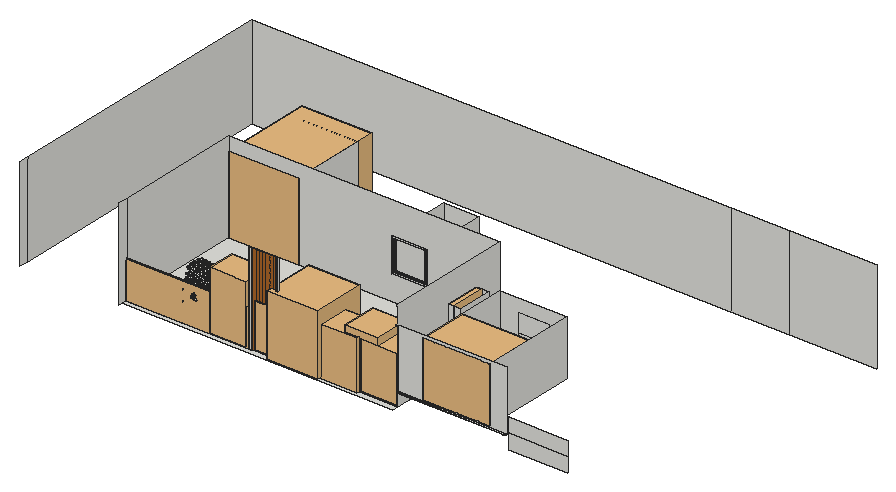
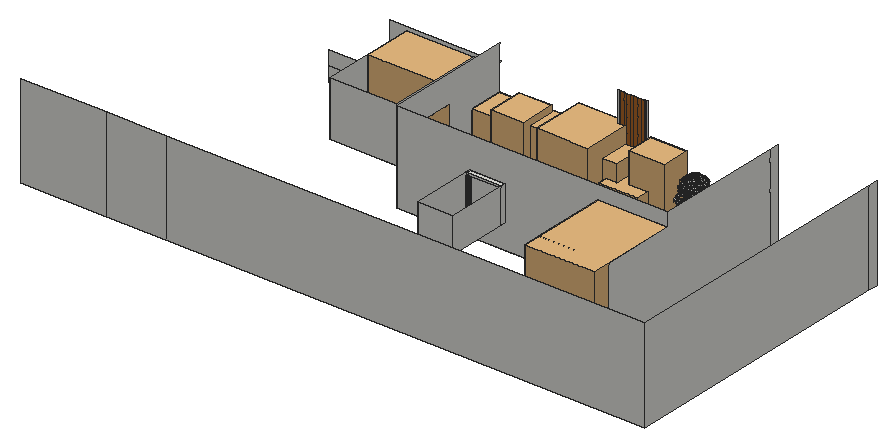
# SketchUp Ruby script. Lengths in inches.
U = 1.inch
M = Sketchup.active_model
def pt(a) = Geom::Point3d.new(a.map { |v| v * U })
def face(e, loops, mat)
  f = e.add_face(loops[0].map { |a| pt(a) })
  loops[1..].each { |l| e.add_face(l.map { |a| pt(a) }).erase! }
  f.material = f.back_material = mat if mat
  f
end
# faces: each face lists its corners as indices into pts; further lists are holes
def faces(e, pts, list, mat = nil) = list.each { |f| face(e, (f[0].is_a?(Array) ? f : [f]).map { |l| l.map { |i| pts[i] } }, mat) }
# xy, xz, yz: faces in a plane at the given z, y or x. An outline is a flat list of corners, or four numbers for a rectangle; further outlines are holes
def ring(l) = l.size == 4 ? [[l[0], l[1]], [l[2], l[1]], [l[2], l[3]], [l[0], l[3]]] : l.each_slice(2).to_a
def flat(e, list, mat, &to3) = list.each { |f| face(e, (f[0].is_a?(Array) ? f : [f]).map { |l| ring(l).map { |u, v| to3.(u, v) } }, mat) }
def xy(e, z, list, mat = nil) = flat(e, list, mat) { |x, y| [x, y, z] }
def xz(e, y, list, mat = nil) = flat(e, list, mat) { |x, z| [x, y, z] }
def yz(e, x, list, mat = nil) = flat(e, list, mat) { |y, z| [x, y, z] }
def lines(e, pts, list) = list.each { |a, b| e.add_line(pt(pts[a]), pt(pts[b])) }
# prism: a flat outline (further loops are holes) pulled along v
def prism(e, loops, v, mat = nil)
  f = face(e, loops, mat); d = Geom::Vector3d.new(v.map { |x| x * U })
  f.pushpull(f.normal.samedirection?(d) ? d.length : -d.length)
end
def box(e, o, s, mat = nil) = prism(e, [[o, [o[0] + s[0], o[1], o[2]], [o[0] + s[0], o[1] + s[1], o[2]], [o[0], o[1] + s[1], o[2]]]], [0, 0, s[2]], mat)
def at(x, y, z, deg = 0) = Geom::Transformation.translation(pt([x, y, z])) * Geom::Transformation.rotation(ORIGIN, Z_AXIS, deg.degrees)
def axes(o, x, y, z) = Geom::Transformation.new([*x, 0, *y, 0, *z, 0, *pt(o).to_a, 1])
def part(name) = M.definitions.add(name)
# library, detail: a bought-in or finely detailed component or shape, given as its bounding box
def library(name, o, s) = part(name).tap { |d| box(d.entities, o, s) }
def detail(e, o, s) = box(e.add_group.entities, o, s)
def put(e, d, t, mat = nil) = e.add_instance(d, t).tap { |i| i.material = mat if mat }
def group(e, t, mat = nil) = e.add_group.tap { |g| g.transformation = t; g.material = mat if mat }.entities
root = M.entities
M.materials.add("[Wood Bamboo]").color = [173, 103, 41]
c1 = library("Glass Railings(black Handrails)",[-57.04,-132.55,0],[169.29,2.52,28.17])
c2 = library("Hanging Plant\#2",[-3.24,-1.74,-0.87],[34.15,22.4,50.98])
c3 = library("Yukka Plant GHD",[0,0,0],[46.13,35.26,75.51])
c4 = library("Philodendron Plant GHD",[-18.43,-10.97,-1.09],[51.75,39.48,62.43])
c5 = library("Plant Banana",[3.49,5.74,0],[38.27,39.55,56.51])
c6 = library("Potted indoor plant",[-35.72,-28.42,0],[66.31,67.39,78.4375])
c7 = part("leaflet")
p = [[2.87,10.24,0.32],[0.33,13.79,0],[-2.24,10.39,0.32],[-2.2,6.92,0.33],[0.45,0.11,0.33],[2.91,6.86,0.33]]
faces(c7.entities,p,[[0,1,2],[0,2,3,4,5]])
c8 = part("leaf group")
put(c8.entities,c7,axes([4.25,4.04,0.04],[0.8,0,0],[0,0.8,0],[0,0,0.8]))
put(c8.entities,c7,axes([4.5,3.78,0.04],[0.4,0.69282,-0.00011],[-0.69282,0.4,-0.00008],[-0.00001,0.00014,0.8]))
put(c8.entities,c7,axes([4.92,3.9375,0.04],[-0.56569,0.56569,-0.00025],[-0.56569,-0.56569,0.00001],[-0.00017,0.00019,0.8]))
put(c8.entities,c7,axes([4.87,4.38,0.04],[-0.69282,-0.4,-0.0002],[0.4,-0.69282,0.00017],[-0.00026,0.00005,0.8]))
put(c8.entities,c7,axes([4.42,4.45,0.04],[0.20706,-0.77274,-0.00003],[0.77274,0.20706,0.00016],[-0.00015,-0.00007,0.8]))
c9 = part("branch with leaves\#1")
put(c9.entities,c8,axes([2.86,31.23,35.15],[-0.02765,-0.79009,-0.61237],[0.48114,-0.54749,0.68465],[-0.8762,-0.27571,0.39528]))
put(c9.entities,c8,axes([12.72,29.5,24.05],[-0.41566,0.90952,0],[-0.44736,-0.20444,-0.87067],[-0.7919,-0.3619,0.49186]))
put(c9.entities,c8,axes([15.91,15.09,15.29],[-0.51919,0.82474,-0.22414],[0.78767,0.35997,-0.5],[-0.33169,-0.43615,-0.83652]))
put(c9.entities,c8,axes([23.4,16.37,17.31],[0.5,0.75,-0.43301],[0,0.5,0.86603],[0.86603,-0.43301,0.25]))
put(c9.entities,c8,axes([11.3125,8.27,23.62],[1.15,0,0],[0,0.575,0.99593],[0,-0.86603,0.5]))
c10 = part("leaflet\#1")
p = [[0.33,13.79,0],[2.87,10.24,0.32],[-2.24,10.39,0.32],[2.91,6.86,0.33],[0.45,0.11,0.33],[-2.2,6.92,0.33]]
faces(c10.entities,p,[[0,1,2],[2,1,3,4,5]])
c11 = part("leaf group\#1")
put(c11.entities,c10,axes([1.8,0.82,0.04],[-0.56569,0.56569,-0.00025],[-0.33941,-0.33941,0.00001],[-0.00017,0.00019,0.8]))
c12 = part("flower")
put(c12.entities,c11,axes([3.87,3.58,0.87],[0.08758,0.98061,-0.17532],[0.93721,-0.14075,-0.31909],[-0.33758,-0.13637,-0.93137]))
put(c12.entities,c11,axes([3.58,5.87,0.87],[0.98061,-0.08758,-0.17532],[-0.14075,-0.93721,-0.31909],[-0.13637,0.33758,-0.93137]))
put(c12.entities,c11,axes([5.87,6.16,0.87],[-0.08758,-0.98061,-0.17532],[-0.93721,0.14075,-0.31909],[0.33758,0.13637,-0.93137]))
put(c12.entities,c11,axes([6.16,3.87,0.87],[-0.98061,0.08758,-0.17532],[0.14075,0.93721,-0.31909],[0.13637,-0.33758,-0.93137]))
put(c12.entities,c11,axes([4.97,4.02,1.64],[-0.54077,0.62855,-0.55902],[0.78035,0.12673,-0.61237],[-0.31406,-0.76738,-0.55902]))
put(c12.entities,c11,axes([4.08,5.2,1.64],[0.81472,0.15405,-0.55902],[-0.28042,-0.73917,-0.61237],[-0.50754,0.65567,-0.55902]))
put(c12.entities,c11,axes([5.55,5.38,1.64],[-0.27395,-0.78259,-0.55902],[-0.49993,0.61243,-0.61237],[0.8216,0.11171,-0.55902]))
c13 = part("branch")
p = [[0.27,0.14,21.6],[1.15,1.36,21.6],[2.31,4.21,0],[0.54,1.79,0],[1.05,2.55,32.4],[1.34,2.95,32.4]]
faces(c13.entities,p,[[0,1,2,3],[4,5,1,0]])
c14 = part("branch with leaves")
put(c14.entities,c8,axes([29.28,4.46,29.75],[0.70711,0.61237,-0.35355],[-0.27393,0.69819,0.66144],[0.65189,-0.37086,0.66144]))
put(c14.entities,c8,axes([2.86,31.23,35.15],[-0.02765,-0.79009,-0.61237],[0.48114,-0.54749,0.68465],[-0.8762,-0.27571,0.39528]))
put(c14.entities,c13,axes([15.22,43.9,5.2],[1,0,0],[0,0.5,0.86603],[0,-1.03923,0.6]))
put(c14.entities,c8,axes([12.72,29.5,24.05],[-0.41566,0.90952,0],[-0.44736,-0.20444,-0.87067],[-0.7919,-0.3619,0.49186]))
put(c14.entities,c8,axes([15.91,15.09,15.29],[-0.51919,0.82474,-0.22414],[0.78767,0.35997,-0.5],[-0.33169,-0.43615,-0.83652]))
put(c14.entities,c8,axes([31.61,42.03,14.23],[-0.02765,-0.79009,-0.61237],[0.47126,0.52995,-0.70503],[0.88156,-0.30808,0.35768]))
put(c14.entities,c8,axes([23.4,16.37,17.31],[0.5,0.75,-0.43301],[0,0.5,0.86603],[0.86603,-0.43301,0.25]))
put(c14.entities,c8,axes([12.04,8.6,24.1875],[1,0,0],[0,0.5,0.86603],[0,-0.86603,0.5]))
c15 = part("trunk")
p = [[2.07,0,0],[2.91,2.57,208.4],[2.76,2.68,208.4],[0.57,1.09,0],[3.93,0,0],[3.09,2.57,208.4],
  [5.43,1.09,0],[3.24,2.68,208.4],[2.7,2.85,208.4],[0,2.85,0],[6,2.85,0],[3.3,2.85,208.4],
  [2.76,3.03,208.4],[0.57,4.62,0],[5.43,4.62,0],[3.24,3.03,208.4],[2.91,3.14,208.4],[2.07,5.71,0],
  [3.93,5.71,0],[3.09,3.14,208.4]]
faces(c15.entities,p,[[0,1,2,3],[4,5,1,0],[6,7,5,4],[3,2,8,9],[6,10,11,7],[8,12,13,9],[11,10,14,15],[13,12,16,17],
  [18,19,15,14],[17,16,19,18]])
c16 = part("Flowering tree")
put(c16.entities,c9,axes([8.5625,69.79,58.85],[-1.14545,-0.10223,0],[0.09875,-1.10642,-0.25882],[0.02646,-0.29646,0.96593]))
put(c16.entities,c12,axes([18.03,-59.9,126.47],[-1.06473,0.02061,0.37747],[-0.32263,-0.80708,-0.6548],[0.29115,-0.81896,0.6548]))
put(c16.entities,c12,axes([24.99,-51.52,163.52],[0.99593,0.2875,-0.43301],[0,0.99593,0.5],[0.575,-0.49796,0.75]))
put(c16.entities,c12,axes([9.15,43.86,180.9375],[-0.776,0.32151,0.68301],[0.59221,-0.55726,0.70711],[0.60796,0.9532,0.18301]))
put(c16.entities,c12,axes([-19.44,51.82,88.4375],[-0.978,0.2192,-0.49033],[-0.25151,-1.12216,0],[-0.55023,0.12332,0.87153]))
put(c16.entities,c9,axes([79.24,-48.01,132.64],[0.21275,1.12031,-0.12941],[-1.10684,0.17595,-0.22414],[-0.22834,0.19092,0.96593]))
put(c16.entities,c9,axes([64.36,-6.43,165.85],[-0.10223,1.14545,0],[-1.10642,-0.09875,-0.25882],[-0.29646,-0.02646,0.96593]))
put(c16.entities,c9,axes([52.57,39.62,163.85],[-0.88224,0.73767,0],[-0.71253,-0.85218,-0.25882],[-0.19092,-0.22834,0.96593]))
put(c16.entities,c9,axes([-64.4,-29.26,175.85],[0.88224,-0.73767,0],[0.71253,0.85218,-0.25882],[0.19092,0.22834,0.96593]))
put(c16.entities,c9,axes([40.35,-16.55,200.81],[-0.14358,1.14093,0.01256],[-0.77283,-0.08933,-0.72016],[-0.83795,-0.11311,0.69546]))
put(c16.entities,c9,axes([7.875,84.56,112.85],[-1.14773,-0.07221,0],[0.06975,-1.10862,-0.25882],[0.01869,-0.29705,0.96593]))
put(c16.entities,c9,axes([-66.42,6.43,163.85],[0.10223,-1.14545,0],[1.10642,0.09875,-0.25882],[0.29646,0.02646,0.96593]))
put(c16.entities,c9,axes([-6.02,-66.82,162.85],[1.14545,0.10223,0],[-0.09875,1.10642,-0.25882],[-0.02646,0.29646,0.96593]))
put(c16.entities,c9,axes([65.22,55.72,70.85],[-0.88224,0.73767,0],[-0.71253,-0.85218,-0.25882],[-0.19092,-0.22834,0.96593]))
put(c16.entities,c9,axes([-6.02,-85.22,100.85],[1.14545,0.10223,0],[-0.09875,1.10642,-0.25882],[-0.02646,0.29646,0.96593]))
put(c16.entities,c9,axes([-64.4,-55.71,70.85],[0.88224,-0.73767,0],[0.71253,0.85218,-0.25882],[0.19092,0.22834,0.96593]))
put(c16.entities,c9,axes([-46.27,-12.7,180.74],[-0.29529,-0.0373,-0.96593],[1.10206,0.13922,-0.25882],[0.14413,-1.14093,0]))
put(c16.entities,c9,axes([56.125,-64.81,70.85],[0.73767,0.88224,0],[-0.85218,0.71253,-0.25882],[-0.22834,0.19092,0.96593]))
put(c16.entities,c9,axes([-55.31,64.8125,78.85],[-0.73767,-0.88224,0],[0.85218,-0.71253,-0.25882],[0.22834,-0.19092,0.96593]))
put(c16.entities,c9,axes([-84.82,6.43,92.85],[0.10223,-1.14545,0],[1.10642,0.09875,-0.25882],[0.29646,0.02646,0.96593]))
put(c16.entities,c14,axes([56.87,3.27,57.34],[-0.44564,1.06014,0],[-1.06014,-0.44564,0],[0,0,1]))
put(c16.entities,c12,axes([-46.02,24.68,176.39],[-0.60389,-0.88348,0.36612],[0.59197,0.06424,0.85552],[-0.77935,0.73337,0.36612]))
put(c16.entities,c14,axes([-18.99,-54,51.28],[1.15,0,0],[0,1.15,0],[0,0,1]))
put(c16.entities,c12,axes([-14.26,69.05,133.89],[-0.21654,-1.04563,0.37124],[1.09634,-0.09014,0.29155],[-0.27139,0.47014,0.88158]))
put(c16.entities,c9,axes([7.875,59.26,173.85],[-1.14773,-0.07221,0],[0.06975,-1.10862,-0.25882],[0.01869,-0.29705,0.96593]))
put(c16.entities,c12,axes([-39.65,-46.59,156.55],[0.81317,-0.40659,0.61237],[0,0.99593,0.5],[-0.81317,-0.40659,0.61237]))
put(c16.entities,c9,axes([68.45,-14.73,133.12],[0.31285,1.10009,0.10445],[-1.0665,0.33304,-0.23681],[-0.29529,-0.0373,0.96593]))
put(c16.entities,c14,axes([-54.71,-13.99,125.23],[0.64805,-0.95001,0],[0.91764,0.62597,-0.25882],[0.24588,0.16773,0.96593]))
put(c16.entities,c12,axes([-59.37,-17.76,103.29],[0.82621,-0.65851,-0.39489],[0.59197,0.06424,0.85552],[-0.538,-0.9406,0.33489]))
put(c16.entities,c14,axes([-55.12,-14.55,89.35],[0.64805,-0.95001,0],[0.91764,0.62597,-0.25882],[0.24588,0.16773,0.96593]))
put(c16.entities,c12,axes([48.53,-28.74,71.58],[0.35234,0.10813,0.94725],[-0.36862,-1.06582,0.19567],[1.03076,-0.41812,-0.25382]))
put(c16.entities,c9,axes([-12.83,63.67,197.61],[0.0612,-1.14229,0.10265],[-1.10726,-0.09004,-0.2585],[0.30453,-0.09784,-0.96054]))
put(c16.entities,c9,axes([-64.4,-55.71,112.85],[0.88224,-0.73767,0],[0.71253,0.85218,-0.25882],[0.19092,0.22834,0.96593]))
put(c16.entities,c9,axes([65.22,55.72,114.85],[-0.88224,0.73767,0],[-0.71253,-0.85218,-0.25882],[-0.19092,-0.22834,0.96593]))
put(c16.entities,c12,axes([63.34,2.95,120.74],[0.8666,0.37799,-0.5693],[-0.45977,1.05409,0],[0.6001,0.26175,0.82213]))
put(c16.entities,c9,axes([85.63,-6.43,94.85],[-0.10223,1.14545,0],[-1.10642,-0.09875,-0.25882],[-0.29646,-0.02646,0.96593]))
put(c16.entities,c14,axes([31.42,47.13,103.94],[-1.11535,0.28016,0],[-0.27473,-1.09373,-0.19595],[-0.0549,-0.21855,0.98061]))
put(c16.entities,c15,axes([-3.39,-3.28,43.76],[1.15,0,0],[0,1.15,0],[0,0,0.79]))
put(c16.entities,c14,axes([34.9,-44.92,95.18],[0.62465,0.96556,0],[-0.93266,0.60337,-0.25882],[-0.24991,0.16167,0.96593]))
put(c16.entities,c14,axes([32.7,-43.8,134.99],[0.62465,0.96556,0],[-0.88615,0.57328,-0.39715],[-0.38347,0.24808,0.91775]))
put(c16.entities,c9,axes([-51.54,49.67,143.57],[0.26379,-0.52212,-0.86096],[0.65423,-0.75347,0.49708],[-0.90824,-0.69439,0.108]))
put(c16.entities,c14,axes([31.48,46.68,140.85],[-1.11535,0.28016,0],[-0.27061,-1.07735,-0.25882],[-0.07251,-0.28867,0.96593]))
put(c16.entities,c9,axes([8.75,19.55,179.21],[-0.27543,0.79346,0.68307],[-1.10726,-0.09004,-0.2585],[-0.14361,-0.82754,0.68307]))
c17 = part("Plant GHD")
put(c17.entities,c16,axes([21.36,20.42,-5.32],[0.2847,0,0],[0,0.2847,0],[0,0,0.33025]))
g1 = group(c17.entities,at(14.85,13.9,0))
detail(g1,[0,0,0],[13.04,13.04,11.8])
c18 = library("Group\#719",[-5.55,-6.67,0],[49.65,49.64,35.75])
c19 = part("Plants indoor GHD")
put(c19.entities,c2,at(254.34,21.02,0))
put(c19.entities,c3,at(45.23,2.59,0))
put(c19.entities,c4,at(201.7,11.53,0))
put(c19.entities,c5,at(99.46,-3.08,1.17))
put(c19.entities,c6,at(158.24,24.68,0))
put(c19.entities,c17,at(0,0,0))
put(c19.entities,c18,at(72.51,10.66,1.17))
c20 = library("Untitled (14)",[0,0,0],[7.13,36,83])
c21 = library("Group\#14",[0,0,0],[39.5,117.4375,51.17])
c22 = library("cay+chuoi",[26.89,19.66,0.52],[41.96,45.65,69.71])
c23 = library("KentiaPalm",[-22.86,-14.31,0],[47.49,43.96,59.125])
c24 = part("Group668\#1")
p = [[0,0,0],[0,0,-13.34],[-3.03,0,-13.34],[19.7,-23.5,0],[-19.7,-23.5,0],[19.7,23.5,0],
  [19.7,0,0],[-19.7,23.5,0],[3.03,0,-13.34],[-19.7,0,0],[0,0,-21.6]]
lines(c24.entities,p,[[0,1],[1,2],[3,4],[5,6],[7,5],[1,8],[9,0],[0,6],[8,10],[4,9],[6,3],[2,10],
  [9,7]])
c25 = part("Rectangle Light")
put(c25.entities,c24,at(0,0,0))
c26 = part("Copyright 2018, ")
xy(c26.entities,0.05,[[[19.06,0,19.06,9.82,21.3125,9.82,22.13,9.76,22.85,9.6,23.48,9.33,24,8.95,24.43,8.48,24.73,7.92,24.91,7.28,24.97,6.54,24.91,5.85,24.74,5.21,24.46,4.64,24.0625,4.14,23.58,3.73,23.03,3.4375,22.42,3.26,21.75,3.2,21.1,3.27,20.375,3.48,20.375,0],[21.62,4.3125,22.05,4.35,22.4375,4.47,22.79,4.66,23.09,4.94,23.34,5.28,23.52,5.66,23.63,6.09,23.67,6.56,23.6,7.16,23.4,7.68,23.08,8.1,22.66,8.39,22.08,8.56,21.28,8.61,20.375,8.61,20.375,4.61,20.98,4.39]],[25.77,0,27.98,4.71,25.47,9.82,26.9375,9.82,28.69,6.14,30.375,9.82,31.82,9.82,27.21,0],[[43.77,0,43.11,0.03,42.52,0.14,41.99,0.3125,41.54,0.55,41.18,0.86,40.92,1.2,40.77,1.6,40.71,2.04,40.82,2.64,41.12,3.13,41.63,3.5,42.35,3.75,41.86,4.16,41.74,4.37,41.7,4.57,41.77,4.87,41.98,5.14,42.3,5.36,42.73,5.51,42.1,5.88,41.65,6.34,41.38,6.91,41.29,7.57,41.34,8.0625,41.48,8.5,41.72,8.88,42.05,9.21,42.47,9.48,42.95,9.67,43.5,9.78,44.13,9.82,46.81,9.82,46.81,8.8125,45.49,8.8125,46.02,8.11,46.13,7.77,46.17,7.38,46.1,6.875,45.88,6.38,45.55,5.94,45.13,5.625,44.53,5.39,43.64,5.21,43.09,5.03,42.96,4.89,42.91,4.71,42.98,4.5,43.18,4.34,44.17,4.04,45.71,3.625,46.33,3.2,46.67,2.67,46.79,2.03,46.74,1.59,46.59,1.2,46.33,0.85,45.97,0.55,45.52,0.31,45.01,0.14,44.42,0.03],[43.74,1.02,44.5,1.09,45.0625,1.28,45.42,1.58,45.53,1.99,45.5,2.2,45.39,2.4,44.94,2.72,44.26,2.9375,43.41,3.01,42.82,2.94,42.34,2.73,42.03,2.42,41.93,2.03,42.04,1.59,42.38,1.28,42.95,1.09],[43.72,6.34,44.22,6.42,44.63,6.67,44.91,7.05,45,7.51,44.9,7.98,44.63,8.36,44.22,8.61,43.71,8.7,43.23,8.61,42.82,8.35,42.54,7.96,42.45,7.5,42.54,7.04,42.8125,6.67,43.22,6.42]],[180.16,0,182.36,4.71,179.85,9.82,181.32,9.82,183.07,6.14,184.75,9.82,186.2,9.82,181.59,0],[[219.8,0,219.13,0.03,218.54,0.14,218.02,0.3125,217.57,0.55,217.21,0.86,216.95,1.2,216.79,1.6,216.74,2.04,216.84,2.64,217.15,3.13,217.66,3.5,218.375,3.75,217.89,4.16,217.77,4.37,217.72,4.57,217.79,4.87,218,5.14,218.33,5.36,218.76,5.51,218.13,5.88,217.68,6.34,217.41,6.91,217.32,7.57,217.37,8.0625,217.51,8.5,217.75,8.88,218.08,9.21,218.5,9.48,218.98,9.67,219.53,9.78,220.16,9.82,222.83,9.82,222.83,8.8125,221.52,8.8125,222.05,8.11,222.16,7.77,222.2,7.38,222.125,6.875,221.91,6.38,221.58,5.94,221.16,5.625,220.5625,5.39,219.67,5.21,219.12,5.03,218.99,4.89,218.94,4.71,219.01,4.5,219.21,4.34,220.2,4.04,221.73,3.625,222.35,3.2,222.7,2.67,222.82,2.03,222.77,1.59,222.61,1.2,222.36,0.85,222,0.55,221.55,0.31,221.03,0.14,220.45,0.03],[219.77,1.02,220.53,1.09,221.09,1.28,221.44,1.58,221.5625,1.99,221.52,2.2,221.41,2.4,220.97,2.72,220.29,2.9375,219.43,3.01,218.84,2.94,218.37,2.73,218.0625,2.42,217.96,2.03,218.07,1.59,218.41,1.28,218.98,1.09],[219.75,6.34,220.25,6.42,220.66,6.67,220.93,7.05,221.02,7.51,220.93,7.98,220.66,8.36,220.24,8.61,219.74,8.7,219.25,8.61,218.85,8.35,218.57,7.96,218.48,7.5,218.57,7.04,218.84,6.67,219.25,6.42]],
  [92.62,1.6,92.62,1.87,92.89,2.17,93.07,2.48,93.22,3.3125,92.89,3.45,92.65,3.66,92.51,3.92,92.47,4.24,92.53,4.6,92.72,4.9,93.01,5.11,93.34,5.18,93.73,5.08,94.04,4.8,94.25,4.36,94.32,3.82,94.2,3.09,93.87,2.45,93.33,1.9375],[6.01,3.2,5.21,3.24,4.48,3.37,3.81,3.58,3.2,3.87,2.66,4.23,2.17,4.66,1.74,5.14,1.38,5.7,1.08,6.29,0.875,6.91,0.75,7.55,0.71,8.22,0.8,9.25,1.09,10.2,1.57,11.07,2.24,11.84,3.06,12.49,3.96,12.95,4.95,13.22,6.04,13.3125,6.83,13.26,7.68,13.11,8.5625,12.86,9.49,12.5,9.49,10.98,8.63,11.42,7.78,11.72,6.9375,11.91,6.11,11.97,5.29,11.9,4.55,11.7,3.89,11.37,3.29,10.9,2.8,10.33,2.45,9.7,2.24,8.99,2.17,8.22,2.24,7.44,2.45,6.74,2.79,6.11,3.27,5.55,3.86,5.09,4.53,4.76,5.27,4.57,6.09,4.5,6.98,4.57,7.87,4.78,8.74,5.12,9.6,5.6,9.6,4.05,8.79,3.68,7.92,3.41,6.99,3.25],[[14.21,3.2,13.51,3.26,12.87,3.4375,12.29,3.73,11.77,4.14,11.34,4.65,11.03,5.21,10.85,5.82,10.78,6.5,10.85,7.1875,11.03,7.81,11.34,8.375,11.78,8.88,12.31,9.3,12.9,9.59,13.55,9.77,14.27,9.83,14.98,9.77,15.63,9.59,16.21,9.29,16.73,8.87,17.16,8.36,17.47,7.79,17.66,7.16,17.72,6.47,17.66,5.79,17.47,5.18,17.16,4.625,16.72,4.13,16.19,3.72,15.6,3.43,14.9375,3.26],[14.25,4.4,14.71,4.44,15.12,4.55,15.48,4.74,15.81,5,16.07,5.32,16.26,5.68,16.37,6.08,16.41,6.53,16.37,6.97,16.25,7.375,16.06,7.74,15.78,8.0625,15.45,8.33,15.07,8.52,14.65,8.63,14.2,8.67,13.76,8.63,13.36,8.52,13,8.33,12.68,8.0625,12.42,7.74,12.23,7.37,12.12,6.97,12.08,6.52,12.12,6.07,12.24,5.67,12.43,5.31,12.69,4.99,13.02,4.73,13.39,4.55,13.8,4.44]],[57.3125,3.2,56.51,3.33,55.84,3.72,55.54,4.07,55.34,4.58,55.26,5.77,55.26,8.66,54.13,8.66,54.13,8.78,56.54,11.16,56.54,9.82,58.6,9.82,58.6,8.66,56.54,8.66,56.54,5.48,56.6,4.99,56.78,4.64,57.06,4.43,57.47,4.36,58.18,4.48,58.93,4.82,58.93,3.62,58.16,3.31],[[88.3125,3.2,87.67,3.25,87.08,3.41,86.54,3.66,86.06,4.02,85.66,4.45,85.37,4.93,85.2,5.46,85.14,6.04,85.23,6.75,85.49,7.37,85.93,7.91,86.54,8.36,86,8.86,85.64,9.37,85.4375,9.91,85.37,10.54,85.43,11.1,85.59,11.61,85.86,12.08,86.24,12.51,86.7,12.86,87.21,13.11,87.76,13.26,88.37,13.3125,88.96,13.26,89.51,13.11,90.01,12.86,90.46,12.51,90.83,12.09,91.09,11.62,91.25,11.1,91.31,10.54,91.23,9.91,91,9.33,90.62,8.82,90.08,8.36,90.68,7.91,91.11,7.38,91.36,6.75,91.45,6.02,91.39,5.4375,91.23,4.91,90.95,4.43,90.56,4,90.08,3.65,89.55,3.4,88.96,3.25],[88.33,4.54,89,4.64,89.54,4.94,89.9,5.39,90.02,5.96,90.02,6.11,89.9,6.72,89.54,7.21,88.98,7.53,88.28,7.64,87.6,7.53,87.05,7.21,86.69,6.71,86.57,6.09,86.69,5.47,87.06,4.98,87.62,4.65],[88.35,9.02,88.95,9.125,89.45,9.45,89.79,9.93,89.9,10.49,89.79,11.08,89.46,11.55,88.96,11.87,88.34,11.97,87.72,11.87,87.22,11.5625,86.89,11.09,86.78,10.51,86.89,9.9375,87.24,9.46,87.75,9.13]],
  [[113.29,3.2,112.92,3.24,112.64,3.36,112.43,3.57,112.32,3.85,111.9,3.57,111.47,3.375,111.03,3.26,110.57,3.22,109.95,3.33,109.44,3.66,109.1,4.17,108.99,4.79,109.1,5.375,109.43,5.89,109.97,6.32,110.6875,6.66,112.33,7.22,112.33,7.57,112.26,8.08,112.04,8.45,111.67,8.67,111.16,8.74,110.64,8.67,110.12,8.47,109.61,8.13,109.11,7.65,109.11,9.06,109.53,9.45,110.02,9.72,110.6,9.89,111.27,9.94,111.77,9.91,112.21,9.81,112.61,9.63,112.95,9.39,113.34,8.92,113.55,8.34,113.6,7.22,113.6,4.46,113.65,4.21,113.82,4.13,114.12,4.21,114.55,4.47,114.55,3.6875,113.85,3.3],[111.19,4.1,111.79,4.22,112.33,4.6,112.33,6.53,111.47,6.2,110.91,5.9375,110.54,5.67,110.34,5.375,110.27,5.01,110.33,4.64,110.53,4.35,110.82,4.16]],[121.02,3.2,120.43,3.28,119.88,3.51,119.43,3.87,119.1,4.34,118.9,5.04,118.83,6.09,118.83,9.82,120.12,9.82,120.12,6.11,120.19,5.24,120.41,4.68,120.82,4.38,121.44,4.28,121.88,4.33,122.29,4.5,122.66,4.78,123,5.17,123,9.82,124.29,9.82,124.29,3.3125,123,3.3125,123,4.15,122.5625,3.75,122.07,3.45,121.54,3.26],[[156.36,3.2,155.99,3.24,155.7,3.36,155.5,3.57,155.39,3.85,154.97,3.57,154.54,3.375,154.1,3.26,153.64,3.22,153.02,3.33,152.51,3.66,152.17,4.17,152.06,4.79,152.17,5.375,152.5,5.89,153.03,6.32,153.75,6.66,155.4,7.22,155.4,7.57,155.33,8.08,155.11,8.45,154.74,8.67,154.23,8.74,153.7,8.67,153.1875,8.47,152.68,8.13,152.18,7.65,152.18,9.06,152.59,9.45,153.09,9.72,153.67,9.89,154.33,9.94,154.83,9.91,155.28,9.81,155.68,9.63,156.02,9.39,156.4,8.92,156.62,8.34,156.66,7.22,156.66,4.46,156.72,4.21,156.89,4.13,157.1875,4.21,157.62,4.47,157.62,3.6875,156.92,3.3],[154.26,4.1,154.85,4.22,155.4,4.6,155.4,6.53,154.54,6.2,153.98,5.9375,153.61,5.67,153.4,5.375,153.34,5.01,153.4,4.64,153.59,4.35,153.89,4.16]],[161.74,3.2,161.01,3.26,160.37,3.43,159.8,3.71,159.3,4.11,158.91,4.6,158.62,5.16,158.45,5.81,158.4,6.53,158.45,7.26,158.62,7.92,158.89,8.5,159.28,9,159.76,9.41,160.3,9.71,160.92,9.88,161.6,9.94,162.51,9.85,163.49,9.49,163.49,8.12,162.55,8.59,161.68,8.74,161.27,8.7,160.89,8.59,160.55,8.4,160.25,8.13,160.01,7.8,159.84,7.4375,159.73,7.02,159.7,6.57,159.73,6.1,159.85,5.68,160.04,5.31,160.3,4.99,160.63,4.73,161.01,4.55,161.44,4.4375,161.93,4.4,162.73,4.51,163.63,4.83,163.63,3.5625,162.67,3.29],[[178.37,3.2,178,3.24,177.71,3.36,177.51,3.57,177.39,3.85,176.98,3.57,176.55,3.375,176.1,3.26,175.65,3.22,175.02,3.33,174.52,3.66,174.18,4.17,174.0625,4.79,174.17,5.375,174.51,5.89,175.04,6.32,175.76,6.66,177.41,7.22,177.41,7.57,177.33,8.08,177.11,8.45,176.75,8.67,176.23,8.74,175.71,8.67,175.19,8.47,174.6875,8.13,174.18,7.65,174.18,9.06,174.6,9.45,175.1,9.72,175.68,9.89,176.34,9.94,176.84,9.91,177.29,9.81,177.68,9.63,178.03,9.39,178.41,8.92,178.625,8.34,178.67,7.22,178.67,4.46,178.73,4.21,178.9,4.13,179.2,4.21,179.625,4.47,179.625,3.6875,178.92,3.3],[176.27,4.1,176.86,4.22,177.41,4.6,177.41,6.53,176.54,6.2,175.98,5.9375,175.61,5.67,175.41,5.375,175.34,5.01,175.41,4.64,175.6,4.35,175.9,4.16]],
  [210.76,3.2,209.73,3.33,208.59,3.78,208.59,5.17,209.71,4.55,210.23,4.37,210.66,4.3125,211.04,4.36,211.36,4.51,211.57,4.73,211.65,4.98,211.6,5.24,211.46,5.45,210.65,5.99,209.62,6.64,209.02,7.18,208.73,7.69,208.64,8.25,208.67,8.6,208.78,8.93,208.96,9.22,209.22,9.47,209.89,9.83,210.72,9.94,211.6875,9.81,212.68,9.41,212.68,8.13,211.64,8.65,210.81,8.83,210.47,8.79,210.2,8.67,210.03,8.48,209.97,8.25,210.02,8.03,210.18,7.82,210.91,7.32,211.37,7.06,212.08,6.59,212.59,6.09,212.89,5.57,213,5.02,212.96,4.64,212.84,4.3,212.64,3.99,212.37,3.71,212.04,3.49,211.66,3.33],[[73.82,3.22,73.14,3.3,72.53,3.56,71.99,3.99,71.52,4.59,71.14,5.34,70.87,6.2,70.7,7.17,70.65,8.25,70.71,9.32,70.875,10.29,71.16,11.15,71.55,11.9,72.03,12.52,72.58,12.96,73.2,13.23,73.88,13.3125,74.53,13.23,75.12,12.96,75.65,12.51,76.125,11.89,76.51,11.13,76.79,10.27,76.96,9.32,77.01,8.28,76.96,7.2,76.79,6.24,76.51,5.38,76.125,4.62,75.65,4.01,75.11,3.57,74.5,3.3],[73.81,4.52,74.2,4.58,74.54,4.77,74.84,5.08,75.1,5.51,75.31,6.06,75.46,6.6875,75.58,8.22,75.46,9.76,75.32,10.4,75.12,10.95,74.87,11.4,74.59,11.72,74.26,11.91,73.89,11.97,73.82,11.97,73.4375,11.91,73.09,11.72,72.79,11.41,72.53,10.97,72.32,10.43,72.18,9.79,72.06,8.26,72.17,6.7,72.32,6.06,72.52,5.51,72.78,5.08,73.08,4.77,73.42,4.58]],[[204.86,3.22,203.89,3.33,203.125,3.66,202.53,4.18,202.06,4.86,201.76,5.67,201.66,6.6,201.71,7.31,201.87,7.95,202.13,8.51,202.5,9.01,202.95,9.42,203.47,9.71,204.05,9.89,204.6875,9.94,205.3,9.89,205.85,9.72,206.33,9.43,206.75,9.04,207.09,8.55,207.33,7.98,207.47,7.34,207.52,6.61,207.52,6.45,202.95,6.45,203.13,5.61,203.32,5.27,203.57,4.97,203.88,4.73,204.23,4.55,205.06,4.42,205.68,4.47,206.28,4.61,206.86,4.86,207.41,5.21,207.41,3.95,206.82,3.61,206.23,3.39,205.6,3.26],[202.98,7.22,206.25,7.22,206.11,7.9,205.79,8.41,205.31,8.72,204.6875,8.83,204.06,8.72,203.55,8.41,203.1875,7.9]],[32.81,3.3125,32.81,9.82,34.1,9.82,34.1,8.33,34.17,8.4375,34.64,9.1,35.1,9.57,35.57,9.85,36.04,9.94,36.4,9.9,36.78,9.76,37.55,9.21,36.875,8.08,36.23,8.55,35.63,8.71,35.33,8.68,35.05,8.57,34.55,8.12,34.21,7.47,34.1,6.71,34.1,3.3125],[38.48,3.3125,39.77,9.82],
  [47.77,3.3125,47.77,13.1875,49.06,13.1875,49.06,8.96,49.49,9.39,49.96,9.7,50.49,9.88,51.06,9.94,51.68,9.86,52.23,9.62,52.68,9.23,52.99,8.72,53.18,8.01,53.24,7.02,53.24,3.3125,51.96,3.3125,51.96,7.34,51.87,7.98,51.61,8.48,51.2,8.81,50.6875,8.92,50.27,8.86,49.89,8.7,49.49,8.41,49.06,7.97,49.06,3.3125],[63.46,3.3125,63.46,3.41,64.06,4.11,66.27,7.04,66.95,8.09,67.35,8.86,67.53,9.47,67.6,10.07,67.48,10.82,67.125,11.41,66.57,11.79,65.87,11.92,65.28,11.83,64.7,11.57,64.15,11.14,63.66,10.58,63.66,12.375,64.24,12.79,64.83,13.08,65.43,13.26,66.04,13.3125,66.65,13.26,67.21,13.1,67.72,12.83,68.17,12.45,68.53,11.99,68.79,11.47,68.95,10.9,69,10.26,68.95,9.65,68.8,8.99,68.51,8.27,68.06,7.4375,67.34,6.4,66.26,5.04,65.95,4.68,69.71,4.68,69.71,3.3125],[80.37,3.3125,81.78,13.1875],[100.21,3.3125,100.21,13.1875,101.625,13.1875,101.625,8.67,105.78,13.1875,107.55,13.1875,103.27,8.5,108.6,3.3125,106.67,3.3125,101.625,8.19,101.625,3.3125],[115.72,3.3125,117,13.1875],
  [126.04,3.3125,126.04,9.82,127.33,9.82,127.33,8.96,127.82,9.39,128.3,9.7,128.78,9.88,129.25,9.94,129.83,9.87,130.35,9.65,130.79,9.28,131.17,8.77,131.6875,9.29,132.22,9.66,132.77,9.88,133.32,9.96,133.77,9.91,134.18,9.78,134.55,9.57,134.88,9.27,135.15,8.875,135.34,8.39,135.45,7.82,135.49,7.15,135.49,3.3125,134.2,3.3125,134.2,7.17,134.12,7.88,133.87,8.41,133.47,8.73,132.92,8.84,132.53,8.79,132.15,8.64,131.78,8.39,131.43,8.04,131.43,3.3125,130.13,3.3125,130.13,6.93,130.0625,7.85,129.84,8.44,129.67,8.63,129.45,8.76,128.83,8.87,128.45,8.82,128.1,8.6875,127.74,8.43,127.33,8.04,127.33,3.3125],[141.43,3.3125,141.43,13.1875,142.77,13.1875,146.05,9.13,149.31,13.1875,150.63,13.1875,150.63,3.3125,149.21,3.3125,149.21,11,146.17,7.18,145.91,7.18,142.84,11,142.84,3.3125],[165.29,3.3125,165.29,13.1875,166.7,13.1875,166.7,8.67,170.86,13.1875,172.62,13.1875,168.34,8.5,173.67,3.3125,171.75,3.3125,166.7,8.19,166.7,3.3125],[214.51,3.3125,215.8,9.82],[223.8,3.3125,223.8,9.82,225.12,9.82,225.12,8.99,225.5625,9.41,226.04,9.7,226.54,9.88,227.07,9.94,227.66,9.86,228.2,9.63,228.67,9.26,229,8.77,229.2,8.06,229.27,7.03,229.27,3.3125,227.99,3.3125,227.99,7.02,227.91,7.87,227.68,8.44,227.28,8.76,226.66,8.87,226.23,8.8125,225.82,8.64,225.45,8.36,225.12,7.96,225.12,3.3125],
  [[191.3125,3.33,191.3125,13.1875,194.64,13.1875,195.6,13.15,196.45,13.04,197.19,12.85,197.83,12.58,198.39,12.25,198.88,11.84,199.32,11.36,199.7,10.81,200,10.21,200.22,9.58,200.35,8.93,200.39,8.25,200.29,7.28,200.01,6.35,199.54,5.5,198.92,4.76,198.14,4.14,197.24,3.7,196.22,3.4,194.4375,3.33],[192.73,4.59,194.54,4.59,195.48,4.62,196.18,4.73,197.16,5.1,197.88,5.65,198.34,6.21,198.66,6.85,198.86,7.55,198.93,8.33,198.86,9.08,198.66,9.77,198.32,10.38,197.85,10.92,197.43,11.26,196.94,11.53,195.97,11.85,194.49,11.93,192.73,11.93]],[39.12,11.03,38.84,11.09,38.59,11.26,38.42,11.51,38.37,11.8,38.42,12.08,38.59,12.32,38.84,12.49,39.12,12.55,39.41,12.5,39.66,12.33,39.83,12.09,39.89,11.8,39.83,11.51,39.66,11.26,39.41,11.09],[215.14,11.03,214.87,11.09,214.62,11.26,214.45,11.51,214.4,11.8,214.45,12.08,214.62,12.32,214.87,12.49,215.14,12.55,215.44,12.5,215.6875,12.33,215.86,12.09,215.92,11.8,215.86,11.51,215.6875,11.26,215.44,11.09]])
xy(root,244.51,[[624.25,908.5,973.0625,908.5,973.0625,997.25,988.8125,997.25,988.8125,1041.93,973.0625,1041.93,973.0625,1080.1875,714.02,1080.1875,714.02,1175.3125,624.25,1175.3125],[782.66,915.1875,785.84,916.1875],[817.03,915.1875,820.03,916.1875]])
xy(root,261.47,[[973.0625,914.15,1112.75,916.1875]])
xy(root,262.47,[[973.0625,914.15,1112.75,916.1875]])
xy(root,263.92,[[1005.21,916.1875,1091.46,1039.625]])
xy(root,276.22,[[834.07,1080.1875,878.82,1086.1875]])
xy(root,276.23,[[834.07,1080.1875,878.82,1163.875]])
xy(root,278.38,[[836.23,1080.1875,876.66,1081.4375],[836.23,1084.9375,876.66,1086.1875]])
xy(root,279.02,[[836.87,1081.4375,876.02,1082.6875],[836.87,1082.6875,876.02,1083.6875],[836.87,1083.6875,876.02,1084.9375]])
xy(root,279.55,[[837.4,1082.6875,875.5,1082.79],[837.4,1082.79,875.5,1083.59],[837.4,1083.59,875.5,1083.6875]])
xy(root,317.65,[[837.4,1082.6875,875.5,1082.79],[837.4,1082.79,875.5,1083.59],[837.4,1083.59,875.5,1083.6875]])
xy(root,318.18,[[836.87,1081.4375,876.02,1082.6875],[836.87,1082.6875,876.02,1083.6875],[836.87,1083.6875,876.02,1084.9375]])
xy(root,318.8125,[[836.23,1080.1875,876.66,1081.4375],[836.23,1084.9375,876.66,1086.1875]])
xy(root,320.98,[[834.07,1080.1875,878.82,1086.1875]])
xy(root,361.64,[[782.66,915.1875,785.84,916.1875],[817.03,915.1875,820.03,916.1875]])
xz(root,914.15,[[973.0625,261.47,1112.75,262.47]])
xz(root,915.1875,[[782.66,244.51,785.84,361.64],[817.03,244.51,820.03,361.64]])
xz(root,916.1875,[[[973.0625,262.47,1112.75,339.08],[1005.21,263.92,1091.46,334.79]]])
xz(root,916.1875,[[785.84,244.51,790.3,361.64],[790.3,244.51,794.75,361.64],[794.75,244.51,799.21,361.64],[799.21,244.51,803.67,361.64],[803.67,244.51,808.12,361.64],
  [808.12,244.51,812.58,361.64],[812.58,244.51,817.03,361.64]],"[Wood Bamboo]")
xz(root,919.75,[[1112.75,242.71,1189.1875,261.31],[1112.75,261.31,1189.1875,279.91]])
xz(root,997.25,[[973.0625,244.51,988.8125,326.83]])
xz(root,1039.625,[[1005.21,263.92,1091.46,334.79]])
xz(root,1041.93,[[973.0625,244.51,988.8125,326.83]])
xz(root,1080.1875,[[[714.02,244.51,973.0625,244.51,973.0625,361.64,624.25,361.64,624.25,344.51,714.02,344.51],[834.07,276.23,878.82,320.98]],[[834.07,276.22,878.82,320.98],[836.23,278.38,876.66,318.8125]]])
xz(root,1081.4375,[[[836.23,278.38,876.66,318.8125],[836.87,279.02,876.02,318.18]]])
xz(root,1082.6875,[[[836.87,279.02,876.02,318.18],[837.4,279.55,875.5,317.65]]])
xz(root,1082.79,[[837.4,279.55,875.5,317.65]])
xz(root,1083.59,[[837.4,279.55,875.5,317.65]])
xz(root,1083.6875,[[[836.87,279.02,876.02,318.18],[837.4,279.55,875.5,317.65]]])
xz(root,1084.9375,[[[836.23,278.38,876.66,318.8125],[836.87,279.02,876.02,318.18]]])
xz(root,1086.1875,[[[834.07,276.22,878.82,320.98],[836.23,278.38,876.66,318.8125]]])
xz(root,1163.875,[[834.07,276.23,878.82,320.98]])
xz(root,1175.3125,[[624.25,244.51,714.02,344.51]])
xz(root,1276.1875,[[497.625,244.51,1112.75,364.51],[1112.75,244.51,1189.1875,364.51],[1189.1875,244.51,1299.8125,364.51]])
yz(root,497.625,[[904.1875,244.51,916.1875,364.51],[916.1875,244.51,1276.1875,364.51]])
yz(root,624.25,[[904.1875,244.51,916.1875,361.64],[916.1875,244.51,1175.3125,244.51,1175.3125,344.51,1080.1875,344.51,1080.1875,361.64,916.1875,361.64]])
yz(root,714.02,[[1080.1875,244.51,1175.3125,344.51]])
yz(root,782.66,[[915.1875,244.51,916.1875,361.64]])
yz(root,785.84,[[915.1875,244.51,916.1875,361.64]],"[Wood Bamboo]")
yz(root,817.03,[[915.1875,244.51,916.1875,361.64]],"[Wood Bamboo]")
yz(root,820.03,[[915.1875,244.51,916.1875,361.64]])
yz(root,834.07,[[1080.1875,276.22,1086.1875,320.98],[1080.1875,276.23,1163.875,320.98]])
yz(root,836.23,[[1080.1875,278.38,1081.4375,318.8125],[1084.9375,278.38,1086.1875,318.8125]])
yz(root,836.87,[[1081.4375,279.02,1082.6875,318.18],[1082.6875,279.02,1083.6875,318.18],[1083.6875,279.02,1084.9375,318.18]])
yz(root,837.4,[[1082.6875,279.55,1082.79,317.65],[1082.79,279.55,1083.59,317.65],[1083.59,279.55,1083.6875,317.65]])
yz(root,875.5,[[1082.6875,279.55,1082.79,317.65],[1082.79,279.55,1083.59,317.65],[1083.59,279.55,1083.6875,317.65]])
yz(root,876.02,[[1081.4375,279.02,1082.6875,318.18],[1082.6875,279.02,1083.6875,318.18],[1083.6875,279.02,1084.9375,318.18]])
yz(root,876.66,[[1080.1875,278.38,1081.4375,318.8125],[1084.9375,278.38,1086.1875,318.8125]])
yz(root,878.82,[[1080.1875,276.22,1086.1875,320.98],[1080.1875,276.23,1163.875,320.98]])
yz(root,973.0625,[[916.1875,244.51,916.1875,261.47,914.15,261.47,914.15,262.47,916.1875,262.47,916.1875,339.08,913.52,339.08,913.52,340.08,916.1875,340.08,916.1875,360.64,915.15,360.64,915.15,361.64,1080.1875,361.64,1080.1875,244.51,1041.93,244.51,1041.93,326.83,997.25,326.83,997.25,244.51]])
yz(root,988.8125,[[997.25,244.51,1041.93,326.83]])
yz(root,1005.21,[[916.1875,263.92,1039.625,334.79]])
yz(root,1091.46,[[916.1875,263.92,1039.625,334.79]])
put(root,c1,axes([677.63,1047.74,244.51],[0.9357,0,0],[0,1,0],[0,0,1.70393]))
put(root,c19,at(687.8,912.24,245.61))
put(root,c20,axes([973.0625,997.25,244.51],[1,0,0],[0,1.24132,0],[0,0,0.99172]))
put(root,c1,axes([871.44,1048.74,244.51],[0.90532,0,0],[0,1,0],[0,0,1.70393]))
put(root,c21,axes([624.35,1080.1875,244.51],[2.27,0,0],[0,1,0],[0,0,1.957]))
put(root,c22,at(877.87,896.53,244.01))
put(root,c23,at(948.17,929.98,246.27))
put(root,c21,axes([1005.38,916.1875,263.92],[2.1792,0,0],[0,0.536,0],[0,0,1.38511]))
put(root,c25,axes([1050.32,1037.49,296.54],[1,0,0],[0,0,-1],[0,1,0]))
put(root,c26,axes([840.86,1084.41,276.22],[0.13928,0,0],[0,-0.1494,0],[0,0,-0.93236]))
